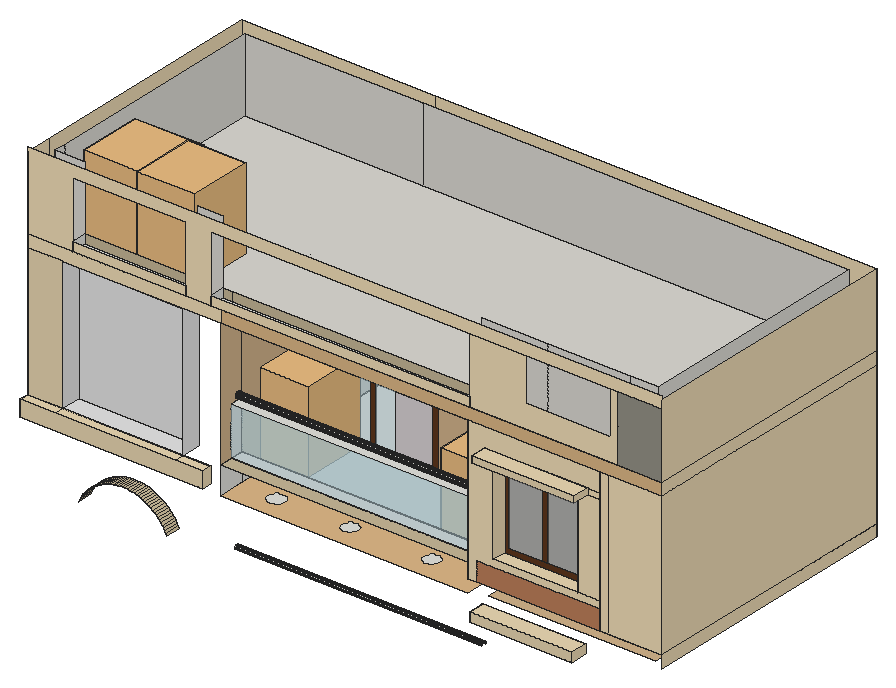
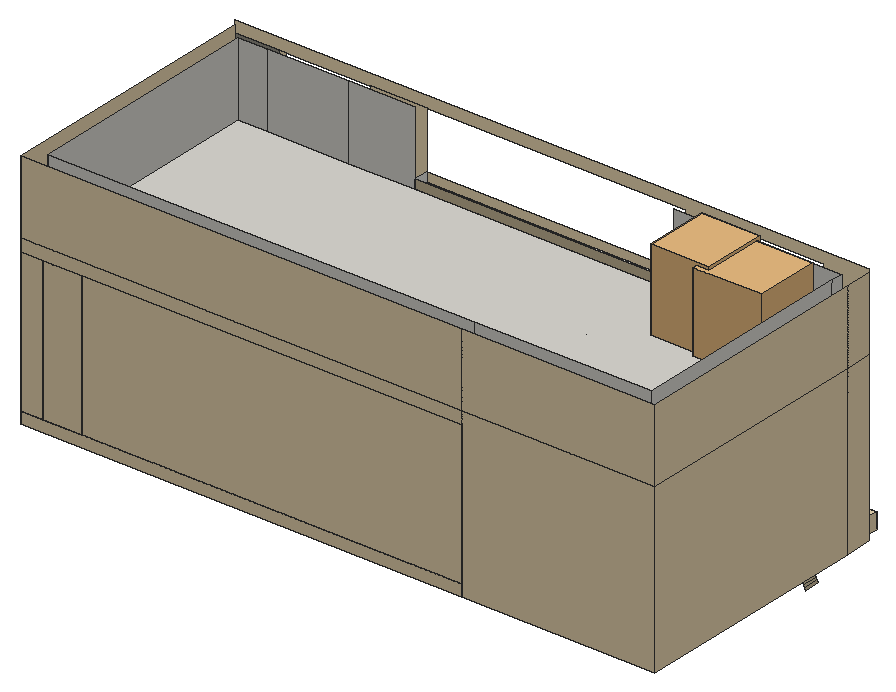
# SketchUp Ruby script. Lengths in inches.
U = 1.inch
M = Sketchup.active_model
def pt(a) = Geom::Point3d.new(a.map { |v| v * U })
def face(e, loops, mat)
  f = e.add_face(loops[0].map { |a| pt(a) })
  loops[1..].each { |l| e.add_face(l.map { |a| pt(a) }).erase! }
  f.material = f.back_material = mat if mat
  f
end
# faces: each face lists its corners as indices into pts; further lists are holes
def faces(e, pts, list, mat = nil) = list.each { |f| face(e, (f[0].is_a?(Array) ? f : [f]).map { |l| l.map { |i| pts[i] } }, mat) }
# xy, xz, yz: faces in a plane at the given z, y or x. An outline is a flat list of corners, or four numbers for a rectangle; further outlines are holes
def ring(l) = l.size == 4 ? [[l[0], l[1]], [l[2], l[1]], [l[2], l[3]], [l[0], l[3]]] : l.each_slice(2).to_a
def flat(e, list, mat, &to3) = list.each { |f| face(e, (f[0].is_a?(Array) ? f : [f]).map { |l| ring(l).map { |u, v| to3.(u, v) } }, mat) }
def xy(e, z, list, mat = nil) = flat(e, list, mat) { |x, y| [x, y, z] }
def xz(e, y, list, mat = nil) = flat(e, list, mat) { |x, z| [x, y, z] }
def yz(e, x, list, mat = nil) = flat(e, list, mat) { |y, z| [x, y, z] }
def lines(e, pts, list) = list.each { |a, b| e.add_line(pt(pts[a]), pt(pts[b])) }
# prism: a flat outline (further loops are holes) pulled along v
def prism(e, loops, v, mat = nil)
  f = face(e, loops, mat); d = Geom::Vector3d.new(v.map { |x| x * U })
  f.pushpull(f.normal.samedirection?(d) ? d.length : -d.length)
end
def box(e, o, s, mat = nil) = prism(e, [[o, [o[0] + s[0], o[1], o[2]], [o[0] + s[0], o[1] + s[1], o[2]], [o[0], o[1] + s[1], o[2]]]], [0, 0, s[2]], mat)
def at(x, y, z, deg = 0) = Geom::Transformation.translation(pt([x, y, z])) * Geom::Transformation.rotation(ORIGIN, Z_AXIS, deg.degrees)
def axes(o, x, y, z) = Geom::Transformation.new([*x, 0, *y, 0, *z, 0, *pt(o).to_a, 1])
def part(name) = M.definitions.add(name)
# library, detail: a bought-in or finely detailed component or shape, given as its bounding box
def library(name, o, s) = part(name).tap { |d| box(d.entities, o, s) }
def detail(e, o, s) = box(e.add_group.entities, o, s)
def put(e, d, t, mat = nil) = e.add_instance(d, t).tap { |i| i.material = mat if mat }
def group(e, t, mat = nil) = e.add_group.tap { |g| g.transformation = t; g.material = mat if mat }.entities
root = M.entities
M.materials.add("[0035_Tan]").color = [210, 180, 140]
M.materials.add("[0036_BurlyWood]").color = [222, 184, 135]
M.materials.add("[Blinds Cellular White]").color = [217, 211, 213]
M.materials.add("[Formica Graystone]").color = [149, 146, 135]
M.materials.add("[Polished Concrete Old]").color = [229, 229, 229]
M.materials.add("[Quartz Light Brown]").color = [242, 223, 185]
M.materials.add("[Quartz Light Brown]1").color = [234, 216, 179]
M.materials.add("[Quartz Light Brown]2").color = [199, 184, 152]
M.materials.add("[Terrazzo Tile Light]").color = [219, 217, 210]
M.materials.add("[Translucent Glass Gray]").color = [128, 128, 128]
M.materials["[Translucent Glass Gray]"].alpha = 0.5
M.materials.add("[Translucent Glass Safety]").color = [204, 235, 244]
M.materials["[Translucent Glass Safety]"].alpha = 0.5
M.materials.add("[Window Covering 02]").color = [199, 178, 115]
M.materials.add("[Wood Veneer 01]").color = [94, 55, 29]
M.materials.add("[Wood Veneer 02]").color = [89, 60, 42]
M.materials.add("[Wood Veneer 02]1").color = [190, 128, 91]
c1 = library("chau cay",[-24.34,-109.24,0],[56.46,62.58,79.69])
c2 = library("Flora+17",[-57.52,158.6,-38.64],[66.99,62.88,77.28])
xy(root,366.625,[[430.17,42.53,593.38,126.3]],"[0035_Tan]")
xy(root,367.28,[[445.44,0,455.38,16.1875],[455.38,0,534.69,16.1875],[534.69,0,545.57,16.1875],[455.38,16.1875,534.69,26.3125]],"[Quartz Light Brown]1")
xy(root,376.66,[[445.44,0,545.57,16.1875]],"[Quartz Light Brown]1")
xy(root,381,[[224.95,31.12,222.83,31.4,220.85,32.22,219.16,33.52,217.86,35.22,217.04,37.19,216.76,39.31,217.04,41.43,217.86,43.4,219.16,45.1,220.85,46.4,222.83,47.22,224.95,47.5,227.07,47.22,229.04,46.4,230.74,45.1,232.04,43.4,232.85,41.43,233.13,39.31,232.85,37.19,232.04,35.22,230.74,33.52,229.04,32.22,227.07,31.4],[297.01,31.12,294.89,31.4,292.91,32.22,291.22,33.52,289.92,35.22,289.1,37.19,288.82,39.31,289.1,41.43,289.92,43.4,291.22,45.1,292.91,46.4,294.89,47.22,297.01,47.5,299.13,47.22,301.1,46.4,302.8,45.1,304.1,43.4,304.92,41.43,305.2,39.31,304.92,37.19,304.1,35.22,302.8,33.52,301.1,32.22,299.13,31.4],[376.7,31.12,374.58,31.4,372.6,32.22,370.91,33.52,369.61,35.22,368.79,37.19,368.51,39.31,368.79,41.43,369.61,43.4,370.91,45.1,372.6,46.4,374.58,47.22,376.7,47.5,378.82,47.22,380.79,46.4,382.49,45.1,383.79,43.4,384.6,41.43,384.88,39.31,384.6,37.19,383.79,35.22,382.49,33.52,380.79,32.22,378.82,31.4]])
xy(root,381,[[[188.57,16.1875,430.17,126.3],[376.7,31.12,378.82,31.4,380.79,32.22,382.49,33.52,383.79,35.22,384.6,37.19,384.88,39.31,384.6,41.43,383.79,43.4,382.49,45.1,380.79,46.4,378.82,47.22,376.7,47.5,374.58,47.22,372.6,46.4,370.91,45.1,369.61,43.4,368.79,41.43,368.51,39.31,368.79,37.19,369.61,35.22,370.91,33.52,372.6,32.22,374.58,31.4],[297.01,31.12,299.13,31.4,301.1,32.22,302.8,33.52,304.1,35.22,304.92,37.19,305.2,39.31,304.92,41.43,304.1,43.4,302.8,45.1,301.1,46.4,299.13,47.22,297.01,47.5,294.89,47.22,292.91,46.4,291.22,45.1,289.92,43.4,289.1,41.43,288.82,39.31,289.1,37.19,289.92,35.22,291.22,33.52,292.91,32.22,294.89,31.4],[224.95,31.12,227.07,31.4,229.04,32.22,230.74,33.52,232.04,35.22,232.85,37.19,233.13,39.31,232.85,41.43,232.04,43.4,230.74,45.1,229.04,46.4,227.07,47.22,224.95,47.5,222.83,47.22,220.85,46.4,219.16,45.1,217.86,43.4,217.04,41.43,216.76,39.31,217.04,37.19,217.86,35.22,219.16,33.52,220.85,32.22,222.83,31.4]]],"[0036_BurlyWood]")
xy(root,387.52,[[0,7.25,34.32,16.1875]])
xy(root,387.52,[[34.32,7.25,151.86,16.1875],[151.86,7.25,178.92,16.1875]],"[Quartz Light Brown]1")
xy(root,393,[[559.62,16.1875,579.5,42.53],[579.5,16.1875,579.5,126.3,597.82,126.3,597.82,278.48,620.12,278.48,620.12,16.1875],[188.57,42.53,559.62,126.3],[559.62,42.53,579.5,126.3],[188.57,126.3,559.62,278.48],
  [559.62,126.3,597.82,278.48]])
xy(root,403.24,[[34.32,16.1875,151.86,35.9375]],"[Polished Concrete Old]")
xy(root,403.24,[[0,7.25,34.32,16.1875],[34.32,7.25,151.86,16.1875],[151.86,7.25,178.92,16.1875]],"[Quartz Light Brown]1")
xy(root,408,[[188.57,29.36,430.17,42.53]])
xy(root,408,[[188.57,16.1875,430.17,29.36]],"[Quartz Light Brown]2")
xy(root,418.73,[[455.23,16.1875,538.1,30.0625]],"[Quartz Light Brown]1")
xy(root,455.875,[[188.57,29.36,430.17,42.53]])
xy(root,507.6,[[446.85,0,547.48,16.1875],[455.23,16.1875,538.1,30.0625]],"[Quartz Light Brown]1")
xy(root,513.74,[[446.85,0,547.48,16.1875]],"[Quartz Light Brown]1")
xy(root,532,[[559.62,16.1875,579.5,126.3],[579.5,16.1875,620.12,126.3],[223.91,36.4,221.63,36.7,219.51,37.58,217.68,38.98,216.28,40.81,215.4,42.93,215.1,45.21,215.4,47.49,216.28,49.62,217.68,51.44,219.51,52.85,221.63,53.73,223.91,54.03,226.19,53.73,228.32,52.85,230.14,51.44,231.54,49.62,232.42,47.49,232.72,45.21,232.42,42.93,231.54,40.81,230.14,38.98,228.32,37.58,226.19,36.7],[303.47,36.4,301.19,36.7,299.07,37.58,297.24,38.98,295.84,40.81,294.96,42.93,294.66,45.21,294.96,47.49,295.84,49.62,297.24,51.44,299.07,52.85,301.19,53.73,303.47,54.03,305.75,53.73,307.88,52.85,309.71,51.44,311.11,49.62,311.99,47.49,312.29,45.21,311.99,42.93,311.11,40.81,309.71,38.98,307.88,37.58,305.75,36.7],[387.72,36.4,385.44,36.7,383.32,37.58,381.49,38.98,380.09,40.81,379.21,42.93,378.91,45.21,379.21,47.49,380.09,49.62,381.49,51.44,383.32,52.85,385.44,53.73,387.72,54.03,390,53.73,392.13,52.85,393.96,51.44,395.36,49.62,396.24,47.49,396.54,45.21,396.24,42.93,395.36,40.81,393.96,38.98,392.13,37.58,390,36.7],
  [559.62,126.3,597.82,278.48],[597.82,126.3,620.12,278.48]])
xy(root,532,[[430.17,16.1875,430.17,126.3,188.57,126.3,188.57,278.48,559.62,278.48,559.62,16.1875]],"[0035_Tan]")
xy(root,532,[[[188.57,16.1875,430.17,126.3],[223.91,36.4,226.19,36.7,228.32,37.58,230.14,38.98,231.54,40.81,232.42,42.93,232.72,45.21,232.42,47.49,231.54,49.62,230.14,51.44,228.32,52.85,226.19,53.73,223.91,54.03,221.63,53.73,219.51,52.85,217.68,51.44,216.28,49.62,215.4,47.49,215.1,45.21,215.4,42.93,216.28,40.81,217.68,38.98,219.51,37.58,221.63,36.7],[387.72,36.4,390,36.7,392.13,37.58,393.96,38.98,395.36,40.81,396.24,42.93,396.54,45.21,396.24,47.49,395.36,49.62,393.96,51.44,392.13,52.85,390,53.73,387.72,54.03,385.44,53.73,383.32,52.85,381.49,51.44,380.09,49.62,379.21,47.49,378.91,45.21,379.21,42.93,380.09,40.81,381.49,38.98,383.32,37.58,385.44,36.7],[303.47,36.4,305.75,36.7,307.88,37.58,309.71,38.98,311.11,40.81,311.99,42.93,312.29,45.21,311.99,47.49,311.11,49.62,309.71,51.44,307.88,52.85,305.75,53.73,303.47,54.03,301.19,53.73,299.07,52.85,297.24,51.44,295.84,49.62,294.96,47.49,294.66,45.21,294.96,42.93,295.84,40.81,297.24,38.98,299.07,37.58,301.19,36.7]]],"[0036_BurlyWood]")
xy(root,532,[[34.32,16.1875,151.86,35.9375]],"[Polished Concrete Old]")
xy(root,544,[[0,16.1875,0,278.48,620.12,278.48,620.12,16.1875,577.38,16.1875,577.38,31.11,605.2,31.11,605.2,263.56,14.92,263.56,14.92,31.11,43.82,31.11,43.82,16.1875],[43.82,16.1875,154.82,31.11],[154.82,16.1875,178.73,31.11],[178.73,16.1875,432.54,31.11],[432.54,16.1875,497.01,31.11],
  [497.01,16.1875,577.38,31.11]])
xy(root,544,[[14.92,31.11,605.2,263.56]],"[Terrazzo Tile Light]")
xz(root,0,[[445.44,367.28,545.57,376.66],[446.85,507.6,547.48,513.74]],"[Quartz Light Brown]1")
xz(root,7.25,[[0,387.52,178.92,403.24]],"[Quartz Light Brown]1")
xz(root,16.1875,[[445.44,367.28,545.57,376.66],[0,387.52,178.92,403.24],[446.85,507.6,547.48,513.74]])
xz(root,16.1875,[[188.57,532,620.12,544]],"[0036_BurlyWood]")
xz(root,16.1875,[[577.38,544,620.12,608.75]],"[Formica Graystone]")
xz(root,16.1875,[[430.17,393,438.87,393,438.87,411.75,559.62,411.75,559.62,418.73,455.23,418.73,455.23,507.6,446.85,507.6,446.85,513.74,559.62,513.74,559.62,532,430.17,532],[559.62,393,567.5,532],[567.5,393,620.12,532],[538.1,418.73,559.62,507.6],[547.48,507.6,559.62,513.74],
  [0,532,188.57,544],[0,544,43.82,544,43.82,608.75,154.82,608.75,154.82,544,178.73,544,178.73,608.75,620.12,608.75,620.12,619.9375,0,619.9375],[43.82,544,154.82,552.75],[178.73,544,432.54,552.75],[432.54,544,577.38,544,577.38,608.75,570.41,608.75,570.41,566.75,486.91,566.75,486.91,608.75,432.54,608.75]],"[Quartz Light Brown]")
xz(root,16.1875,[[0,403.24,34.32,532]],"[Quartz Light Brown]1")
xz(root,16.1875,[[438.87,393,559.62,411.75]],"[Wood Veneer 02]1")
xz(root,29.36,[[188.57,408,430.17,455.875]],"[Translucent Glass Safety]")
xz(root,30.0625,[[459.95,423.45,492.55,502.88],[498.04,423.45,533.38,502.88]],"[Translucent Glass Gray]")
xz(root,30.0625,[[[455.23,418.73,538.1,507.6],[459.95,423.45,533.38,502.88]],[492.55,423.45,498.04,502.88]],"[Wood Veneer 01]")
xz(root,31.11,[[43.82,544,154.82,552.75],[178.73,544,188.57,552.75],[188.57,544,432.54,552.75]],"[Quartz Light Brown]2")
xz(root,31.11,[[14.92,544,43.82,616],[154.82,544,178.73,616],[432.54,544,497.01,616],[497.01,544,577.38,616],[577.38,544,605.2,616]],"[Terrazzo Tile Light]")
xz(root,35.9375,[[34.32,403.24,151.86,532]],"[Polished Concrete Old]")
xz(root,42.53,[[188.57,393,430.17,408],[430.17,393,579.5,520.75]])
xz(root,42.53,[[188.57,408,430.17,455.875]],"[Translucent Glass Safety]")
xz(root,126.3,[[579.5,393,597.82,532]])
xz(root,126.3,[[[188.57,393,207.85,393,207.85,519.0625,314.1,519.0625,314.1,393,579.5,393,579.5,520.75,430.17,520.75,430.17,532,188.57,532],[340.375,471.18,380.5625,524.11]]],"[0035_Tan]")
xz(root,126.3,[[214.22,399.37,230.64,512.69],[272.37,399.37,307.73,512.69]],"[Blinds Cellular White]")
xz(root,126.3,[[230.64,399.37,247.07,512.69],[252.38,399.37,272.37,512.69]],"[Translucent Glass Safety]")
xz(root,126.3,[[334.37,331.34,357.43,367.03],[346.75,477.55,374.19,517.74]],"[Window Covering 02]")
xz(root,126.3,[[[207.85,393,314.1,519.0625],[214.22,399.37,307.73,512.69]],[247.07,399.37,252.38,512.69]],"[Wood Veneer 01]")
xz(root,126.3,[[[329.65,326.625,362.15,371.75],[334.37,331.34,357.43,367.03]],[[340.375,471.18,380.5625,524.11],[346.75,477.55,374.19,517.74]]],"[Wood Veneer 02]")
xz(root,263.56,[[14.92,544,188.57,616],[188.57,544,605.2,616]],"[Terrazzo Tile Light]")
xz(root,278.48,[[0,381,188.57,544],[188.57,381,620.12,393],[188.57,393,559.62,532],[559.62,393,597.82,532],[597.82,393,620.12,532],
  [188.57,532,620.12,544],[0,544,188.57,616],[188.57,544,620.12,616]],"[Quartz Light Brown]1")
yz(root,0,[[16.1875,381,42.53,544],[42.53,381,278.48,544],[7.25,387.52,16.1875,403.24],[16.1875,544,42.53,616],[42.53,544,278.48,616]],"[Quartz Light Brown]1")
yz(root,14.92,[[31.11,544,42.53,616],[42.53,544,263.56,616]],"[Terrazzo Tile Light]")
yz(root,34.32,[[16.1875,403.24,35.9375,532]],"[Polished Concrete Old]")
yz(root,43.82,[[16.1875,544,31.11,552.75]])
yz(root,151.86,[[16.1875,403.24,35.9375,532]],"[Polished Concrete Old]")
yz(root,154.82,[[16.1875,544,31.11,552.75]])
yz(root,178.73,[[16.1875,544,31.11,552.75]])
yz(root,178.92,[[7.25,387.52,16.1875,403.24]],"[Quartz Light Brown]1")
yz(root,188.57,[[16.1875,381,42.53,408],[42.53,381,126.3,393],[126.3,381,278.48,393],[126.3,393,278.48,532],[29.36,408,42.53,455.875]])
yz(root,188.57,[[42.53,393,126.3,532],[[16.1875,408,29.36,408,29.36,455.875,42.53,455.875,42.53,532,16.1875,532],[36.58,457.99,35.84,458.08,35.15,458.37,34.55,458.83,34.09,459.42,33.81,460.12,33.71,460.86,33.81,461.61,34.09,462.3,34.55,462.89,35.15,463.35,35.84,463.64,36.58,463.74,37.33,463.64,38.02,463.35,38.62,462.89,39.07,462.3,39.36,461.61,39.46,460.86,39.36,460.12,39.07,459.42,38.62,458.83,38.02,458.37,37.33,458.08]]],"[0035_Tan]")
yz(root,430.17,[[16.1875,393,42.53,408],[29.36,408,42.53,455.875],[36.58,457.99,37.33,458.08,38.02,458.37,38.62,458.83,39.07,459.42,39.36,460.12,39.46,460.86,39.36,461.61,39.07,462.3,38.62,462.89,38.02,463.35,37.33,463.64,36.58,463.74,35.84,463.64,35.15,463.35,34.55,462.89,34.09,462.3,33.81,461.61,33.71,460.86,33.81,460.12,34.09,459.42,34.55,458.83,35.15,458.37,35.84,458.08]])
yz(root,430.17,[[[16.1875,408,16.1875,532,126.3,532,126.3,520.75,42.53,520.75,42.53,455.875,29.36,455.875,29.36,408],[36.58,457.99,37.33,458.08,38.02,458.37,38.62,458.83,39.07,459.42,39.36,460.12,39.46,460.86,39.36,461.61,39.07,462.3,38.62,462.89,38.02,463.35,37.33,463.64,36.58,463.74,35.84,463.64,35.15,463.35,34.55,462.89,34.09,462.3,33.81,461.61,33.71,460.86,33.81,460.12,34.09,459.42,34.55,458.83,35.15,458.37,35.84,458.08]]],"[0035_Tan]")
yz(root,432.54,[[16.1875,544,31.11,552.75]])
yz(root,445.44,[[0,376.22,16.1875,376.66]])
yz(root,445.44,[[0,367.28,16.1875,376.22]],"[Quartz Light Brown]1")
yz(root,446.85,[[0,507.6,16.1875,513.74]],"[Quartz Light Brown]1")
yz(root,455.23,[[16.1875,418.73,30.0625,507.6]],"[Quartz Light Brown]1")
yz(root,538.1,[[16.1875,418.73,30.0625,507.6]],"[Quartz Light Brown]1")
yz(root,545.57,[[0,367.28,16.1875,376.66]],"[Quartz Light Brown]1")
yz(root,547.48,[[0,507.6,16.1875,513.74]],"[Quartz Light Brown]1")
yz(root,559.62,[[16.1875,393,278.48,532]],"[0035_Tan]")
yz(root,597.82,[[126.3,393,278.48,532]])
yz(root,605.2,[[31.11,544,263.56,616]],"[Terrazzo Tile Light]")
yz(root,620.12,[[16.1875,381,278.48,393],[16.1875,393,278.48,532],[16.1875,532,278.48,544],[16.1875,544,278.48,616]],"[Quartz Light Brown]1")
p = [[430.17,34.01,326.62],[430.17,33.93,327.17],[188.57,33.93,327.17],[188.57,34.01,326.62],[430.17,38.18,327.17],[430.17,38.11,326.62],
  [188.57,38.11,326.62],[188.57,38.18,327.17],[50.61,16.1875,329.04],[49.6,16.1875,327],[49.6,30.875,327],[50.61,30.875,329.04],
  [136.57,16.1875,327],[135.57,16.1875,329.04],[135.57,30.875,329.04],[136.57,30.875,327],[430.17,34.01,327.72],[188.57,34.01,327.72],
  [430.17,38.11,327.72],[188.57,38.11,327.72],[430.17,34.22,328.23],[188.57,34.22,328.23],[430.17,37.9,328.23],[188.57,37.9,328.23],
  [430.17,34.56,328.67],[188.57,34.56,328.67],[430.17,37.5625,328.67],[188.57,37.5625,328.67],[430.17,35,329.01],[188.57,35,329.01],
  [430.17,37.12,329.01],[188.57,37.12,329.01],[51.7,16.1875,331.03],[51.7,30.875,331.03],[134.48,16.1875,331.03],[134.48,30.875,331.03],
  [430.17,35.51,329.22],[188.57,35.51,329.22],[430.17,36.61,329.22],[188.57,36.61,329.22],[430.17,36.06,329.29],[188.57,36.06,329.29],
  [52.89,16.1875,332.96],[52.89,30.875,332.96],[133.29,16.1875,332.96],[133.29,30.875,332.96],[54.17,16.1875,334.84],[54.17,30.875,334.84],
  [132.01,16.1875,334.84],[132.01,30.875,334.84],[55.54,16.1875,336.65],[55.54,30.875,336.65],[130.64,16.1875,336.65],[130.64,30.875,336.65],
  [56.99,16.1875,338.4],[56.99,30.875,338.4],[129.19,16.1875,338.4],[129.19,30.875,338.4],[58.52,16.1875,340.08],[58.52,30.875,340.08],
  [127.66,16.1875,340.08],[127.66,30.875,340.08],[60.13,16.1875,341.68],[60.13,30.875,341.68],[126.05,16.1875,341.68],[126.05,30.875,341.68],
  [61.82,16.1875,343.2],[61.82,30.875,343.2],[124.36,16.1875,343.2],[124.36,30.875,343.2],[63.57,16.1875,344.64],[63.57,30.875,344.64],
  [122.61,16.1875,344.64],[122.61,30.875,344.64],[65.39,16.1875,346],[65.39,30.875,346],[120.78,16.1875,346],[120.78,30.875,346],
  [67.28,16.1875,347.27],[67.28,30.875,347.27],[118.9,16.1875,347.27],[118.9,30.875,347.27],[69.22,16.1875,348.45],[69.22,30.875,348.45],
  [116.96,16.1875,348.45],[116.96,30.875,348.45],[71.21,16.1875,349.53],[71.21,30.875,349.53],[114.96,16.1875,349.53],[114.96,30.875,349.53],
  [73.26,16.1875,350.52],[73.26,30.875,350.52],[112.92,16.1875,350.52],[112.92,30.875,350.52],[75.35,16.1875,351.41],[75.35,30.875,351.41],
  [110.83,16.1875,351.41],[110.83,30.875,351.41],[77.48,16.1875,352.2],[77.48,30.875,352.2],[108.7,16.1875,352.2],[108.7,30.875,352.2],
  [79.64,16.1875,352.89],[79.64,30.875,352.89],[106.54,16.1875,352.89],[106.54,30.875,352.89],[81.84,16.1875,353.48],[81.84,30.875,353.48],
  [104.34,16.1875,353.48],[104.34,30.875,353.48],[84.06,16.1875,353.96],[84.06,30.875,353.96],[102.12,16.1875,353.96],[102.12,30.875,353.96],
  [86.3,16.1875,354.34],[86.3,30.875,354.34],[99.88,16.1875,354.34],[99.88,30.875,354.34],[88.55,16.1875,354.61],[88.55,30.875,354.61],
  [97.625,16.1875,354.61],[97.625,30.875,354.61],[90.82,16.1875,354.77],[90.82,30.875,354.77],[95.36,16.1875,354.77],[95.36,30.875,354.77],
  [93.09,16.1875,354.82],[93.09,30.875,354.82],[430.17,36.58,457.99],[430.17,35.84,458.08],[188.57,35.84,458.08],[188.57,36.58,457.99],
  [430.17,37.33,458.08],[188.57,37.33,458.08],[430.17,35.15,458.37],[188.57,35.15,458.37],[430.17,38.02,458.37],[188.57,38.02,458.37],
  [430.17,34.55,458.83],[188.57,34.55,458.83],[430.17,38.62,458.83],[188.57,38.62,458.83],[430.17,34.09,459.42],[188.57,34.09,459.42],
  [430.17,39.07,459.42],[188.57,39.07,459.42],[430.17,33.81,460.12],[188.57,33.81,460.12],[430.17,39.36,460.12],[188.57,39.36,460.12],
  [430.17,33.71,460.86],[188.57,33.71,460.86],[430.17,39.46,460.86],[188.57,39.46,460.86],[430.17,33.81,461.61],[188.57,33.81,461.61],
  [430.17,39.36,461.61],[188.57,39.36,461.61],[430.17,34.09,462.3],[188.57,34.09,462.3],[430.17,39.07,462.3],[188.57,39.07,462.3],
  [430.17,34.55,462.89],[188.57,34.55,462.89],[430.17,38.62,462.89],[188.57,38.62,462.89],[430.17,35.15,463.35],[188.57,35.15,463.35],
  [430.17,38.02,463.35],[188.57,38.02,463.35],[430.17,35.84,463.64],[188.57,35.84,463.64],[430.17,37.33,463.64],[188.57,37.33,463.64],
  [430.17,36.58,463.74],[188.57,36.58,463.74],[593.38,126.3,366.625],[593.38,126.3,381],[188.57,42.53,532],[188.57,42.53,544],
  [188.57,126.3,532],[188.57,126.3,544],[620.12,126.3,381]]
faces(root,p,[[0,1,2,3],[4,5,6,7],[1,16,17,2],[18,4,7,19],[16,20,21,17],[22,18,19,23],[20,24,25,21],[26,22,23,27],
  [24,28,29,25],[30,26,27,31],[28,36,37,29],[38,30,31,39],[36,40,41,37],[40,38,39,41],[128,129,130,131],[132,128,131,133],
  [129,134,135,130],[136,132,133,137],[134,138,139,135],[140,136,137,141],[138,142,143,139],[144,140,141,145],[142,146,147,143],[148,144,145,149],
  [146,150,151,147],[152,148,149,153],[150,154,155,151],[156,152,153,157],[154,158,159,155],[160,156,157,161],[158,162,163,159],[164,160,161,165],
  [162,166,167,163],[168,164,165,169],[166,170,171,167],[172,168,169,173],[170,174,175,171],[174,172,173,175]],"[Terrazzo Tile Light]")
faces(root,p,[[8,9,10,11],[12,13,14,15],[32,8,11,33],[13,34,35,14],[42,32,33,43],[34,44,45,35],[46,42,43,47],[44,48,49,45],
  [50,46,47,51],[48,52,53,49],[54,50,51,55],[52,56,57,53],[58,54,55,59],[56,60,61,57],[62,58,59,63],[60,64,65,61],
  [66,62,63,67],[64,68,69,65],[70,66,67,71],[68,72,73,69],[74,70,71,75],[72,76,77,73],[78,74,75,79],[76,80,81,77],
  [82,78,79,83],[80,84,85,81],[86,82,83,87],[84,88,89,85],[90,86,87,91],[88,92,93,89],[94,90,91,95],[92,96,97,93],
  [98,94,95,99],[96,100,101,97],[102,98,99,103],[100,104,105,101],[106,102,103,107],[104,108,109,105],[110,106,107,111],[108,112,113,109],
  [114,110,111,115],[112,116,117,113],[118,114,115,119],[116,120,121,117],[122,118,119,123],[120,124,125,121],[126,122,123,127],[124,126,127,125]],"[Quartz Light Brown]2")
lines(root,p,[[176,177],[178,179],[180,181],[177,182]])
put(root,c1,at(399.92,160.98,393))
put(root,c1,at(204.76,172.96,393))
put(root,c1,at(117.45,142.64,544))
put(root,c2,at(95.15,-120.79,582.64))
